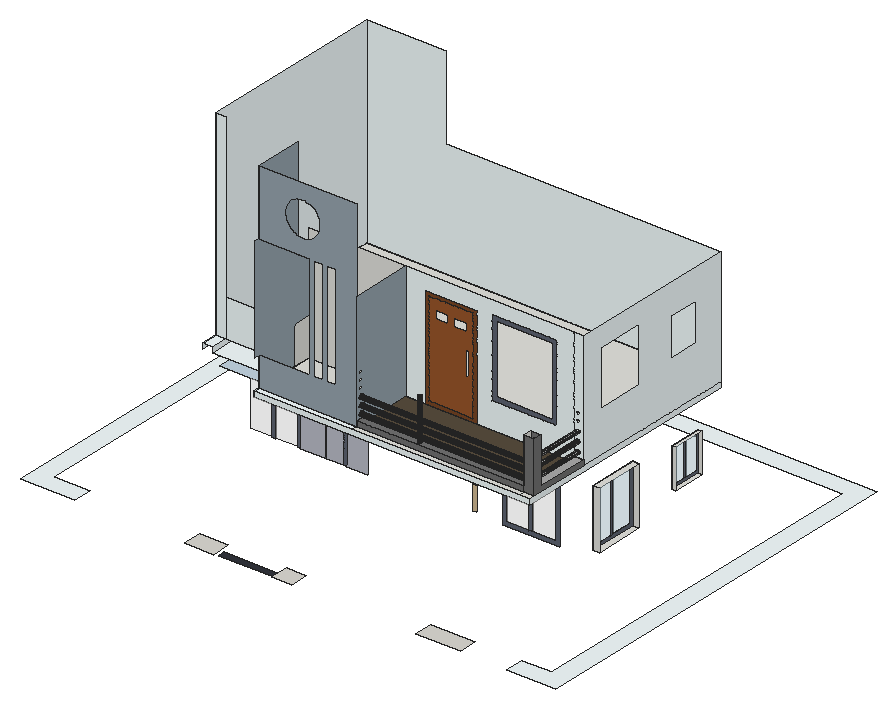
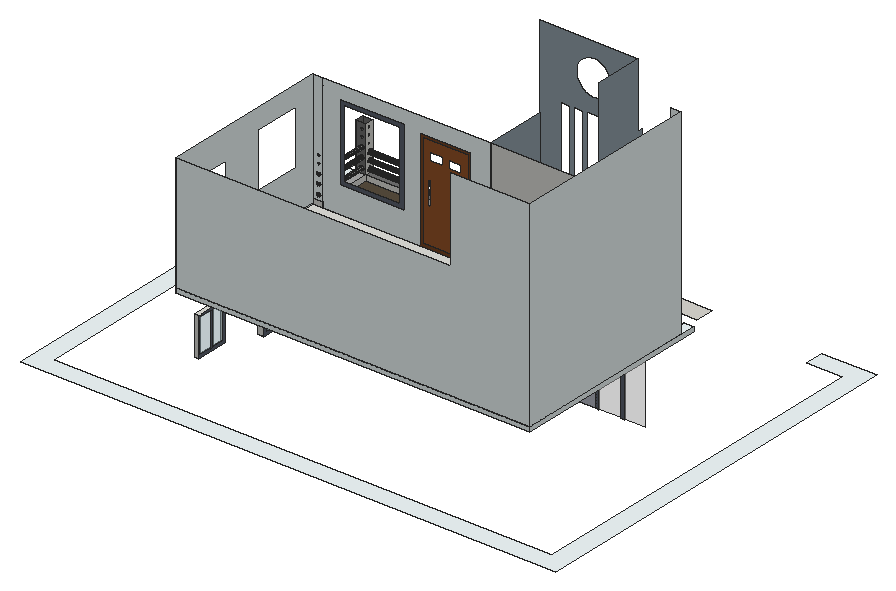
# SketchUp Ruby script. Lengths in inches.
U = 1.inch
M = Sketchup.active_model
def pt(a) = Geom::Point3d.new(a.map { |v| v * U })
def face(e, loops, mat)
  f = e.add_face(loops[0].map { |a| pt(a) })
  loops[1..].each { |l| e.add_face(l.map { |a| pt(a) }).erase! }
  f.material = f.back_material = mat if mat
  f
end
# faces: each face lists its corners as indices into pts; further lists are holes
def faces(e, pts, list, mat = nil) = list.each { |f| face(e, (f[0].is_a?(Array) ? f : [f]).map { |l| l.map { |i| pts[i] } }, mat) }
# xy, xz, yz: faces in a plane at the given z, y or x. An outline is a flat list of corners, or four numbers for a rectangle; further outlines are holes
def ring(l) = l.size == 4 ? [[l[0], l[1]], [l[2], l[1]], [l[2], l[3]], [l[0], l[3]]] : l.each_slice(2).to_a
def flat(e, list, mat, &to3) = list.each { |f| face(e, (f[0].is_a?(Array) ? f : [f]).map { |l| ring(l).map { |u, v| to3.(u, v) } }, mat) }
def xy(e, z, list, mat = nil) = flat(e, list, mat) { |x, y| [x, y, z] }
def xz(e, y, list, mat = nil) = flat(e, list, mat) { |x, z| [x, y, z] }
def yz(e, x, list, mat = nil) = flat(e, list, mat) { |y, z| [x, y, z] }
def lines(e, pts, list) = list.each { |a, b| e.add_line(pt(pts[a]), pt(pts[b])) }
# prism: a flat outline (further loops are holes) pulled along v
def prism(e, loops, v, mat = nil)
  f = face(e, loops, mat); d = Geom::Vector3d.new(v.map { |x| x * U })
  f.pushpull(f.normal.samedirection?(d) ? d.length : -d.length)
end
def box(e, o, s, mat = nil) = prism(e, [[o, [o[0] + s[0], o[1], o[2]], [o[0] + s[0], o[1] + s[1], o[2]], [o[0], o[1] + s[1], o[2]]]], [0, 0, s[2]], mat)
def at(x, y, z, deg = 0) = Geom::Transformation.translation(pt([x, y, z])) * Geom::Transformation.rotation(ORIGIN, Z_AXIS, deg.degrees)
def axes(o, x, y, z) = Geom::Transformation.new([*x, 0, *y, 0, *z, 0, *pt(o).to_a, 1])
def part(name) = M.definitions.add(name)
# library, detail: a bought-in or finely detailed component or shape, given as its bounding box
def library(name, o, s) = part(name).tap { |d| box(d.entities, o, s) }
def detail(e, o, s) = box(e.add_group.entities, o, s)
def put(e, d, t, mat = nil) = e.add_instance(d, t).tap { |i| i.material = mat if mat }
def group(e, t, mat = nil) = e.add_group.tap { |g| g.transformation = t; g.material = mat if mat }.entities
root = M.entities
M.materials.add("[Blinds Roman Hobbled Blue]").color = [187, 189, 201]
M.materials.add("[Carpet Diamond Olive]").color = [87, 77, 61]
M.materials.add("[Color M03]").color = [170, 170, 170]
M.materials.add("[Color M05]").color = [114, 114, 114]
M.materials.add("[Formica Beige]").color = [211, 187, 149]
M.materials.add("[Formica Graystone]").color = [229, 224, 207]
M.materials.add("[Formica Laminate Dark]").color = [95, 101, 114]
M.materials.add("[Formica Laminate Dark]1").color = [50, 53, 60]
M.materials.add("[Terrazzo Light Blue]").color = [151, 165, 175]
M.materials.add("[Terrazzo Light Blue]1").color = [196, 214, 227]
M.materials.add("[Terrazzo Tile Light]").color = [219, 217, 210]
M.materials.add("[Translucent Glass Gray]").color = [242, 242, 242]
M.materials["[Translucent Glass Gray]"].alpha = 0.5
M.materials.add("[Translucent Glass Safety]").color = [204, 235, 244]
M.materials["[Translucent Glass Safety]"].alpha = 0.5
M.materials.add("[White Subway Tile]").color = [243, 252, 253]
M.materials.add("[White Subway Tile]1").color = [243, 252, 253]
M.materials.add("[Wood Cherry Original]").color = [152, 86, 42]
M.materials.add("[Wood Veneer 01]").color = [120, 70, 37]
xy(root,402.23,[[1357.59,44.85,1765.91,92.78]],"[Formica Laminate Dark]1")
xy(root,402.84,[[2922.36,1375.57,2968.68,1724.7]])
xy(root,429.3125,[[1157.35,0,1357.59,129.42],[1765.91,0,1905.75,129.42],[2778.47,0,3092.67,129.42]],"[Terrazzo Tile Light]")
xy(root,429.3125,[[0,0,383.65,0,383.65,129.42,129.42,129.42,129.42,2686.64,3633.2,2686.64,3633.2,129.42,3421.78,129.42,3421.78,0,3762.625,0,3762.625,2816.0625,0,2816.0625]],"[White Subway Tile]1")
xy(root,498.46,[[2941.74,2046.63,2968.68,2278.38]])
xy(root,771.33,[[2941.74,2046.63,2968.68,2278.38]])
xy(root,809.34,[[2922.36,1375.57,2968.68,1724.7]])
xy(root,905.79,[[594.7,1008.89,1485.01,1239.01]],"[Terrazzo Light Blue]1")
xy(root,973.375,[[1034.97,761.77,1522.59,1008.89],[1522.59,761.77,1717.43,803.71],[2898.76,761.77,2968.68,803.71],[1034.97,1008.89,1522.59,1008.89,1522.59,1933.89,547.35,1933.89,547.35,1239.01,1034.97,1239.01],[1717.43,1239.01,2898.76,1933.89]])
xy(root,973.375,[[1717.43,761.77,2898.76,1239.01]],"[Terrazzo Light Blue]1")
xy(root,973.375,[[547.35,1008.89,1034.97,1239.01]],"[White Subway Tile]")
xy(root,1009.375,[[1720.33,761.77,2898.76,803.71],[2898.76,761.77,2968.68,803.71],[1034.97,803.71,1720.33,1239.01],[1720.33,803.71,1720.33,859.31,2898.76,859.31,2898.76,1239.01,2968.68,1239.01,2968.68,803.71],[477.43,1118.14,477.43,2442.87,2968.68,2442.87,2968.68,1239.01,547.35,1239.01,547.35,1118.14],
  [547.35,1118.14,1034.97,1239.01]])
xy(root,1009.375,[[1720.33,859.31,2898.76,1239.01]],"[Carpet Diamond Olive]")
xy(root,1009.375,[[1034.97,761.77,1720.33,803.71],[477.43,1008.89,547.35,1118.14]],"[White Subway Tile]")
xy(root,1046.4375,[[2140.61,820.84,2137.6,821.24,2134.79,822.4,2132.39,824.25,2130.54,826.66,2129.38,829.46,2128.98,832.47,2129.38,835.48,2130.54,838.28,2132.39,840.69,2134.79,842.54,2137.6,843.7,2140.61,844.09,2143.62,843.7,2146.42,842.54,2148.83,840.69,2150.67,838.28,2151.84,835.48,2152.23,832.47,2151.84,829.46,2150.67,826.66,2148.83,824.25,2146.42,822.4,2143.62,821.24]])
xy(root,1046.4375,[[2898.76,859.31,2968.68,1239.01]],"[Color M03]")
xy(root,1046.4375,[[[1720.33,803.71,2898.76,859.31],[2140.61,820.84,2137.6,821.24,2134.79,822.4,2132.39,824.25,2130.54,826.66,2129.38,829.46,2128.98,832.47,2129.38,835.48,2130.54,838.28,2132.39,840.69,2134.79,842.54,2137.6,843.7,2140.61,844.09,2143.62,843.7,2146.42,842.54,2148.83,840.69,2150.67,838.28,2151.84,835.48,2152.23,832.47,2151.84,829.46,2150.67,826.66,2148.83,824.25,2146.42,822.4,2143.62,821.24]]],"[Color M05]")
xz(root,761.77,[[1034.97,973.375,2968.68,1009.375]],"[White Subway Tile]")
xz(root,803.71,[[1720.33,1009.375,2898.76,1046.4375],[2898.76,1009.375,2968.68,1369.75]],"[Color M05]")
xz(root,803.71,[[[1034.97,1009.375,1720.33,1009.375,1720.33,2410.6875,1034.97,2410.6875,1034.97,1949.53,1389.66,1949.53,1389.66,1217.33,1034.97,1217.33],[1341.18,2057.61,1328.27,2058.29,1315.51,2060.3125,1303.02,2063.66,1290.95,2068.29,1279.43,2074.16,1268.59,2081.2,1258.55,2089.33,1249.4,2098.47,1241.27,2108.52,1234.23,2119.36,1228.36,2130.88,1223.73,2142.95,1220.38,2155.43,1218.36,2168.2,1217.68,2181.11,1218.36,2194.02,1220.38,2206.79,1223.73,2219.28,1228.36,2231.34,1234.23,2242.86,1241.27,2253.7,1249.4,2263.75,1258.55,2272.89,1268.59,2281.03,1279.43,2288.07,1290.95,2293.93,1303.02,2298.57,1315.51,2301.91,1328.27,2303.94,1341.18,2304.61,1354.09,2303.94,1366.86,2301.91,1379.35,2298.57,1391.42,2293.93,1402.93,2288.07,1413.77,2281.03,1423.82,2272.89,1432.96,2263.75,1441.1,2253.7,1448.14,2242.86,1454.01,2231.34,1458.64,2219.28,1461.98,2206.79,1464.01,2194.02,1464.68,2181.11,1464.01,2168.2,1461.98,2155.43,1458.64,2142.95,1454.01,2130.88,1448.14,2119.36,1441.1,2108.52,1432.96,2098.47,1423.82,2089.33,1413.77,2081.2,1402.93,2074.16,1391.42,2068.29,1379.35,2063.66,1366.86,2060.3125,1354.09,2058.29],[1421.94,1217.36,1482.63,1947.36],[1511.44,1217.36,1572.13,1947.36]]],"[Terrazzo Light Blue]")
xz(root,859.31,[[1720.33,1009.375,2898.76,1046.4375],[2927.58,1067.59,2930.84,1068.02,2933.87,1069.27,2936.47,1071.27,2938.46,1073.87,2939.72,1076.9,2940.15,1080.15,2939.72,1083.4,2938.46,1086.43,2936.47,1089.03,2933.87,1091.03,2930.84,1092.29,2927.58,1092.71,2924.33,1092.29,2921.3,1091.03,2918.7,1089.03,2916.7,1086.43,2915.45,1083.4,2915.02,1080.15,2915.45,1076.9,2916.7,1073.87,2918.7,1071.27,2921.3,1069.27,2924.33,1068.02],[2927.58,1135.59,2930.84,1136.02,2933.87,1137.27,2936.47,1139.27,2938.46,1141.87,2939.72,1144.9,2940.15,1148.15,2939.72,1151.4,2938.46,1154.43,2936.47,1157.03,2933.87,1159.03,2930.84,1160.29,2927.58,1160.71,2924.33,1160.29,2921.3,1159.03,2918.7,1157.03,2916.7,1154.43,2915.45,1151.4,2915.02,1148.15,2915.45,1144.9,2916.7,1141.87,2918.7,1139.27,2921.3,1137.27,2924.33,1136.02],[2927.58,1200.78,2930.84,1201.2,2933.87,1202.46,2936.47,1204.46,2938.46,1207.06,2939.72,1210.09,2940.15,1213.34,2939.72,1216.59,2938.46,1219.62,2936.47,1222.22,2933.87,1224.22,2930.84,1225.47,2927.58,1225.9,2924.33,1225.47,2921.3,1224.22,2918.7,1222.22,2916.7,1219.62,2915.45,1216.59,2915.02,1213.34,2915.45,1210.09,2916.7,1207.06,2918.7,1204.46,2921.3,1202.46,2924.33,1201.2]])
xz(root,859.31,[[[2898.76,1046.4375,2968.68,1369.75],[2927.58,1316.03,2930.84,1316.45,2933.87,1317.71,2936.47,1319.71,2938.46,1322.31,2939.72,1325.34,2940.15,1328.59,2939.72,1331.84,2938.46,1334.87,2936.47,1337.47,2933.87,1339.47,2930.84,1340.72,2927.58,1341.15,2924.33,1340.72,2921.3,1339.47,2918.7,1337.47,2916.7,1334.87,2915.45,1331.84,2915.02,1328.59,2915.45,1325.34,2916.7,1322.31,2918.7,1319.71,2921.3,1317.71,2924.33,1316.45],[2927.58,1067.59,2930.84,1068.02,2933.87,1069.27,2936.47,1071.27,2938.46,1073.87,2939.72,1076.9,2940.15,1080.15,2939.72,1083.4,2938.46,1086.43,2936.47,1089.03,2933.87,1091.03,2930.84,1092.29,2927.58,1092.71,2924.33,1092.29,2921.3,1091.03,2918.7,1089.03,2916.7,1086.43,2915.45,1083.4,2915.02,1080.15,2915.45,1076.9,2916.7,1073.87,2918.7,1071.27,2921.3,1069.27,2924.33,1068.02],[2927.58,1264.46,2930.84,1264.89,2933.87,1266.15,2936.47,1268.14,2938.46,1270.75,2939.72,1273.77,2940.15,1277.03,2939.72,1280.28,2938.46,1283.31,2936.47,1285.91,2933.87,1287.91,2930.84,1289.16,2927.58,1289.59,2924.33,1289.16,2921.3,1287.91,2918.7,1285.91,2916.7,1283.31,2915.45,1280.28,2915.02,1277.03,2915.45,1273.77,2916.7,1270.75,2918.7,1268.14,2921.3,1266.15,2924.33,1264.89],[2927.58,1135.59,2930.84,1136.02,2933.87,1137.27,2936.47,1139.27,2938.46,1141.87,2939.72,1144.9,2940.15,1148.15,2939.72,1151.4,2938.46,1154.43,2936.47,1157.03,2933.87,1159.03,2930.84,1160.29,2927.58,1160.71,2924.33,1160.29,2921.3,1159.03,2918.7,1157.03,2916.7,1154.43,2915.45,1151.4,2915.02,1148.15,2915.45,1144.9,2916.7,1141.87,2918.7,1139.27,2921.3,1137.27,2924.33,1136.02],[2927.58,1200.78,2930.84,1201.2,2933.87,1202.46,2936.47,1204.46,2938.46,1207.06,2939.72,1210.09,2940.15,1213.34,2939.72,1216.59,2938.46,1219.62,2936.47,1222.22,2933.87,1224.22,2930.84,1225.47,2927.58,1225.9,2924.33,1225.47,2921.3,1224.22,2918.7,1222.22,2916.7,1219.62,2915.45,1216.59,2915.02,1213.34,2915.45,1210.09,2916.7,1207.06,2918.7,1204.46,2921.3,1202.46,2924.33,1201.2]]],"[Color M05]")
xz(root,1118.14,[[477.43,1009.375,547.35,2410.6875],[547.35,1009.375,1034.97,1272.1]],"[White Subway Tile]")
xz(root,1239.01,[[547.35,973.375,1034.97,1009.375],[1034.97,1009.375,1720.33,1828.125],[2898.76,1009.375,2968.68,1046.4375]])
xz(root,1239.01,[[981.69,419.96,1149.58,873.24],[1165.1875,419.96,1280.47,873.24],[1305.85,419.96,1452.47,873.24]],"[Blinds Roman Hobbled Blue]")
xz(root,1239.01,[[2190.67,454.58,2217.05,620.33]],"[Formica Beige]")
xz(root,1239.01,[[2125.16,693.23,2217.66,761.05],[1985.88,705.68,2074.875,760.68]],"[Formica Graystone]")
xz(root,1239.01,[[778.16,419.96,803.87,873.24],[957.16,419.96,981.69,873.24],[1149.58,419.96,1165.1875,873.24],[1280.47,419.96,1305.85,873.24],[[2398.08,439.46,2800.45,879.09],[2425.17,466.55,2773.37,852]],
  [2585.66,466.55,2609.16,852],[[2322.55,1192.6,2780.61,1737.72],[2353.98,1224.02,2749.1875,1706.3]]],"[Formica Laminate Dark]")
xz(root,1239.01,[[627.24,419.96,778.16,873.24],[803.87,419.96,957.16,873.24],[2425.17,466.55,2585.66,852],[2609.16,466.55,2773.37,852]],"[Translucent Glass Gray]")
xz(root,1239.01,[[[1720.33,1009.375,1856.64,1009.375,1856.64,1722.125,2215.15,1722.125,2215.15,1009.375,2898.76,1009.375,2898.76,1828.125,1720.33,1828.125],[2322.55,1192.6,2780.61,1737.72]],[[2898.76,1046.4375,2968.68,1828.125],[2927.58,1316.03,2924.33,1316.45,2921.3,1317.71,2918.7,1319.71,2916.7,1322.31,2915.45,1325.34,2915.02,1328.59,2915.45,1331.84,2916.7,1334.87,2918.7,1337.47,2921.3,1339.47,2924.33,1340.72,2927.58,1341.15,2930.84,1340.72,2933.87,1339.47,2936.47,1337.47,2938.46,1334.87,2939.72,1331.84,2940.15,1328.59,2939.72,1325.34,2938.46,1322.31,2936.47,1319.71,2933.87,1317.71,2930.84,1316.45],[2927.58,1264.46,2924.33,1264.89,2921.3,1266.15,2918.7,1268.14,2916.7,1270.75,2915.45,1273.77,2915.02,1277.03,2915.45,1280.28,2916.7,1283.31,2918.7,1285.91,2921.3,1287.91,2924.33,1289.16,2927.58,1289.59,2930.84,1289.16,2933.87,1287.91,2936.47,1285.91,2938.46,1283.31,2939.72,1280.28,2940.15,1277.03,2939.72,1273.77,2938.46,1270.75,2936.47,1268.14,2933.87,1266.15,2930.84,1264.89],[2927.58,1200.78,2924.33,1201.2,2921.3,1202.46,2918.7,1204.46,2916.7,1207.06,2915.45,1210.09,2915.02,1213.34,2915.45,1216.59,2916.7,1219.62,2918.7,1222.22,2921.3,1224.22,2924.33,1225.47,2927.58,1225.9,2930.84,1225.47,2933.87,1224.22,2936.47,1222.22,2938.46,1219.62,2939.72,1216.59,2940.15,1213.34,2939.72,1210.09,2938.46,1207.06,2936.47,1204.46,2933.87,1202.46,2930.84,1201.2],[2927.58,1135.59,2924.33,1136.02,2921.3,1137.27,2918.7,1139.27,2916.7,1141.87,2915.45,1144.9,2915.02,1148.15,2915.45,1151.4,2916.7,1154.43,2918.7,1157.03,2921.3,1159.03,2924.33,1160.29,2927.58,1160.71,2930.84,1160.29,2933.87,1159.03,2936.47,1157.03,2938.46,1154.43,2939.72,1151.4,2940.15,1148.15,2939.72,1144.9,2938.46,1141.87,2936.47,1139.27,2933.87,1137.27,2930.84,1136.02],[2927.58,1067.59,2924.33,1068.02,2921.3,1069.27,2918.7,1071.27,2916.7,1073.87,2915.45,1076.9,2915.02,1080.15,2915.45,1083.4,2916.7,1086.43,2918.7,1089.03,2921.3,1091.03,2924.33,1092.29,2927.58,1092.71,2930.84,1092.29,2933.87,1091.03,2936.47,1089.03,2938.46,1086.43,2939.72,1083.4,2940.15,1080.15,2939.72,1076.9,2938.46,1073.87,2936.47,1071.27,2933.87,1069.27,2930.84,1068.02]]],"[White Subway Tile]")
xz(root,1239.01,[[[1880.3,1033.03,2191.5,1698.47],[1925.5625,1566.2,2014.55,1621.2],[2058.375,1566.2,2147.37,1621.2],[2136.34,1281.23,2162.72,1446.98]]],"[Wood Cherry Original]")
xz(root,1239.01,[[[1856.64,1009.375,2215.15,1722.125],[1880.3,1033.03,2191.5,1698.47]]],"[Wood Veneer 01]")
xz(root,1375.57,[[2922.36,402.84,2968.68,809.34]])
xz(root,1724.7,[[2922.36,402.84,2968.68,809.34]])
xz(root,2046.63,[[2941.74,498.46,2968.68,771.33]])
xz(root,2278.38,[[2941.74,498.46,2968.68,771.33]])
xz(root,2442.87,[[477.43,973.375,2968.68,1009.375],[477.43,1009.375,477.43,2410.6875,1034.97,2410.6875,1034.97,1828.125,2968.68,1828.125,2968.68,1009.375]],"[White Subway Tile]")
yz(root,477.43,[[1008.89,973.375,2442.87,1009.375],[1118.14,1009.375,2442.87,2410.6875]],"[White Subway Tile]")
yz(root,547.35,[[1008.89,973.375,1239.01,1009.375]],"[White Subway Tile]")
yz(root,1034.97,[[1118.14,1009.375,1239.01,1272.1]])
yz(root,1034.97,[[803.71,1009.375,803.71,1217.33,767.89,1217.33,767.89,1949.53,803.71,1949.53,803.71,2410.6875,1146.14,2410.6875,1146.14,1690.66,1239.01,1690.66,1239.01,1272.1,1118.14,1272.1,1118.14,1009.375]],"[Terrazzo Light Blue]")
yz(root,1034.97,[[761.77,973.375,1239.01,1009.375]],"[White Subway Tile]")
yz(root,1720.33,[[803.71,1009.375,859.31,1046.4375]])
yz(root,1720.33,[[[859.31,1009.375,1239.01,1009.375,1239.01,1828.125,803.71,1828.125,803.71,1046.4375,859.31,1046.4375],[834.19,1325.79,830.94,1326.22,827.91,1327.47,825.3125,1329.47,823.32,1332.07,822.06,1335.1,821.63,1338.35,822.06,1341.6,823.32,1344.63,825.3125,1347.24,827.91,1349.23,830.94,1350.49,834.19,1350.92,837.45,1350.49,840.48,1349.23,843.08,1347.24,845.07,1344.63,846.33,1341.6,846.76,1338.35,846.33,1335.1,845.07,1332.07,843.08,1329.47,840.48,1327.47,837.45,1326.22],[834.19,1277.73,830.94,1278.16,827.91,1279.41,825.3125,1281.41,823.32,1284.01,822.06,1287.04,821.63,1290.29,822.06,1293.54,823.32,1296.57,825.3125,1299.17,827.91,1301.17,830.94,1302.43,834.19,1302.85,837.45,1302.43,840.48,1301.17,843.08,1299.17,845.07,1296.57,846.33,1293.54,846.76,1290.29,846.33,1287.04,845.07,1284.01,843.08,1281.41,840.48,1279.41,837.45,1278.16],[834.19,1224.6,830.94,1225.03,827.91,1226.29,825.3125,1228.28,823.32,1230.88,822.06,1233.91,821.63,1237.17,822.06,1240.42,823.32,1243.45,825.3125,1246.05,827.91,1248.05,830.94,1249.3,834.19,1249.73,837.45,1249.3,840.48,1248.05,843.08,1246.05,845.07,1243.45,846.33,1240.42,846.76,1237.17,846.33,1233.91,845.07,1230.88,843.08,1228.28,840.48,1226.29,837.45,1225.03],[834.19,1172.92,830.94,1173.34,827.91,1174.6,825.3125,1176.6,823.32,1179.2,822.06,1182.23,821.63,1185.48,822.06,1188.73,823.32,1191.76,825.3125,1194.36,827.91,1196.36,830.94,1197.61,834.19,1198.04,837.45,1197.61,840.48,1196.36,843.08,1194.36,845.07,1191.76,846.33,1188.73,846.76,1185.48,846.33,1182.23,845.07,1179.2,843.08,1176.6,840.48,1174.6,837.45,1173.34],[834.19,1120.17,830.94,1120.59,827.91,1121.85,825.3125,1123.85,823.32,1126.45,822.06,1129.48,821.63,1132.73,822.06,1135.98,823.32,1139.01,825.3125,1141.61,827.91,1143.61,830.94,1144.86,834.19,1145.29,837.45,1144.86,840.48,1143.61,843.08,1141.61,845.07,1139.01,846.33,1135.98,846.76,1132.73,846.33,1129.48,845.07,1126.45,843.08,1123.85,840.48,1121.85,837.45,1120.59],[834.19,1065.04,830.94,1065.47,827.91,1066.72,825.3125,1068.72,823.32,1071.32,822.06,1074.35,821.63,1077.6,822.06,1080.85,823.32,1083.88,825.3125,1086.49,827.91,1088.48,830.94,1089.74,834.19,1090.17,837.45,1089.74,840.48,1088.48,843.08,1086.49,845.07,1083.88,846.33,1080.85,846.76,1077.6,846.33,1074.35,845.07,1071.32,843.08,1068.72,840.48,1066.72,837.45,1065.47]]],"[Terrazzo Light Blue]")
yz(root,2898.76,[[859.31,1009.375,1239.01,1046.4375],[[803.71,1046.4375,859.31,1369.75],[834.19,1325.79,837.45,1326.22,840.48,1327.47,843.08,1329.47,845.07,1332.07,846.33,1335.1,846.76,1338.35,846.33,1341.6,845.07,1344.63,843.08,1347.24,840.48,1349.23,837.45,1350.49,834.19,1350.92,830.94,1350.49,827.91,1349.23,825.3125,1347.24,823.32,1344.63,822.06,1341.6,821.63,1338.35,822.06,1335.1,823.32,1332.07,825.3125,1329.47,827.91,1327.47,830.94,1326.22],[834.19,1065.04,837.45,1065.47,840.48,1066.72,843.08,1068.72,845.07,1071.32,846.33,1074.35,846.76,1077.6,846.33,1080.85,845.07,1083.88,843.08,1086.49,840.48,1088.48,837.45,1089.74,834.19,1090.17,830.94,1089.74,827.91,1088.48,825.3125,1086.49,823.32,1083.88,822.06,1080.85,821.63,1077.6,822.06,1074.35,823.32,1071.32,825.3125,1068.72,827.91,1066.72,830.94,1065.47],[834.19,1277.73,837.45,1278.16,840.48,1279.41,843.08,1281.41,845.07,1284.01,846.33,1287.04,846.76,1290.29,846.33,1293.54,845.07,1296.57,843.08,1299.17,840.48,1301.17,837.45,1302.43,834.19,1302.85,830.94,1302.43,827.91,1301.17,825.3125,1299.17,823.32,1296.57,822.06,1293.54,821.63,1290.29,822.06,1287.04,823.32,1284.01,825.3125,1281.41,827.91,1279.41,830.94,1278.16],[834.19,1120.17,837.45,1120.59,840.48,1121.85,843.08,1123.85,845.07,1126.45,846.33,1129.48,846.76,1132.73,846.33,1135.98,845.07,1139.01,843.08,1141.61,840.48,1143.61,837.45,1144.86,834.19,1145.29,830.94,1144.86,827.91,1143.61,825.3125,1141.61,823.32,1139.01,822.06,1135.98,821.63,1132.73,822.06,1129.48,823.32,1126.45,825.3125,1123.85,827.91,1121.85,830.94,1120.59],[834.19,1224.6,837.45,1225.03,840.48,1226.29,843.08,1228.28,845.07,1230.88,846.33,1233.91,846.76,1237.17,846.33,1240.42,845.07,1243.45,843.08,1246.05,840.48,1248.05,837.45,1249.3,834.19,1249.73,830.94,1249.3,827.91,1248.05,825.3125,1246.05,823.32,1243.45,822.06,1240.42,821.63,1237.17,822.06,1233.91,823.32,1230.88,825.3125,1228.28,827.91,1226.29,830.94,1225.03],[834.19,1172.92,837.45,1173.34,840.48,1174.6,843.08,1176.6,845.07,1179.2,846.33,1182.23,846.76,1185.48,846.33,1188.73,845.07,1191.76,843.08,1194.36,840.48,1196.36,837.45,1197.61,834.19,1198.04,830.94,1197.61,827.91,1196.36,825.3125,1194.36,823.32,1191.76,822.06,1188.73,821.63,1185.48,822.06,1182.23,823.32,1179.2,825.3125,1176.6,827.91,1174.6,830.94,1173.34]],[834.19,1065.04,837.45,1065.47,840.48,1066.72,843.08,1068.72,845.07,1071.32,846.33,1074.35,846.76,1077.6,846.33,1080.85,845.07,1083.88,843.08,1086.49,840.48,1088.48,837.45,1089.74,834.19,1090.17,830.94,1089.74,827.91,1088.48,825.3125,1086.49,823.32,1083.88,822.06,1080.85,821.63,1077.6,822.06,1074.35,823.32,1071.32,825.3125,1068.72,827.91,1066.72,830.94,1065.47],[834.19,1120.17,837.45,1120.59,840.48,1121.85,843.08,1123.85,845.07,1126.45,846.33,1129.48,846.76,1132.73,846.33,1135.98,845.07,1139.01,843.08,1141.61,840.48,1143.61,837.45,1144.86,834.19,1145.29,830.94,1144.86,827.91,1143.61,825.3125,1141.61,823.32,1139.01,822.06,1135.98,821.63,1132.73,822.06,1129.48,823.32,1126.45,825.3125,1123.85,827.91,1121.85,830.94,1120.59],[834.19,1172.92,837.45,1173.34,840.48,1174.6,843.08,1176.6,845.07,1179.2,846.33,1182.23,846.76,1185.48,846.33,1188.73,845.07,1191.76,843.08,1194.36,840.48,1196.36,837.45,1197.61,834.19,1198.04,830.94,1197.61,827.91,1196.36,825.3125,1194.36,823.32,1191.76,822.06,1188.73,821.63,1185.48,822.06,1182.23,823.32,1179.2,825.3125,1176.6,827.91,1174.6,830.94,1173.34]])
yz(root,2922.36,[[[1375.57,402.84,1724.7,809.34],[1394.9,422.17,1705.37,790.01]],[1537.67,422.17,1555.72,790.01]],"[Formica Laminate Dark]")
yz(root,2922.36,[[1394.9,422.17,1537.67,790.01],[1555.72,422.17,1705.37,790.01]],"[Translucent Glass Safety]")
yz(root,2941.74,[[[2046.63,498.46,2278.38,771.33],[2064.02,515.84,2261,753.95]],[2153.63,515.84,2169.77,753.95]],"[Formica Laminate Dark]")
yz(root,2941.74,[[2064.02,515.84,2153.63,753.95],[2169.77,515.84,2261,753.95]],"[Translucent Glass Safety]")
yz(root,2968.68,[[803.71,1009.375,1239.01,1009.375,1239.01,1046.4375,859.31,1046.4375,859.31,1369.75,803.71,1369.75]],"[Color M05]")
yz(root,2968.68,[[761.77,973.375,2442.87,1009.375],[[1239.01,1009.375,2442.87,1828.125],[1390.76,1302.22,1726.13,1686.6],[2002.64,1348.11,2223.02,1615.93]]],"[White Subway Tile]")
p = [[2137.6,821.24,1046.4375],[2140.61,820.84,1046.4375],[2140.61,820.84,1339.25],[2137.6,821.24,1339.25],[2143.62,821.24,1046.4375],[2143.62,821.24,1339.25],
  [2134.79,822.4,1046.4375],[2134.79,822.4,1339.25],[2146.42,822.4,1046.4375],[2146.42,822.4,1339.25],[2132.39,824.25,1046.4375],[2132.39,824.25,1339.25],
  [2148.83,824.25,1046.4375],[2148.83,824.25,1339.25],[2130.54,826.66,1046.4375],[2130.54,826.66,1339.25],[2150.67,826.66,1046.4375],[2150.67,826.66,1339.25],
  [2129.38,829.46,1046.4375],[2129.38,829.46,1339.25],[2151.84,829.46,1046.4375],[2151.84,829.46,1339.25],[2128.98,832.47,1046.4375],[2128.98,832.47,1339.25],
  [2152.23,832.47,1046.4375],[2152.23,832.47,1339.25],[2129.38,835.48,1046.4375],[2129.38,835.48,1339.25],[2151.84,835.48,1046.4375],[2151.84,835.48,1339.25],
  [2130.54,838.28,1046.4375],[2130.54,838.28,1339.25],[2150.67,838.28,1046.4375],[2150.67,838.28,1339.25],[2132.39,840.69,1046.4375],[2132.39,840.69,1339.25],
  [2148.83,840.69,1046.4375],[2148.83,840.69,1339.25],[2134.79,842.54,1046.4375],[2134.79,842.54,1339.25],[2146.42,842.54,1046.4375],[2146.42,842.54,1339.25],
  [2137.6,843.7,1046.4375],[2137.6,843.7,1339.25],[2143.62,843.7,1046.4375],[2143.62,843.7,1339.25],[2140.61,844.09,1046.4375],[2140.61,844.09,1339.25],
  [2898.76,834.19,1065.04],[2898.76,830.94,1065.47],[1720.33,830.94,1065.47],[1720.33,834.19,1065.04],[2898.76,837.45,1065.47],[1720.33,837.45,1065.47],
  [2898.76,827.91,1066.72],[1720.33,827.91,1066.72],[2898.76,840.48,1066.72],[1720.33,840.48,1066.72],[2898.76,825.3125,1068.72],[1720.33,825.3125,1068.72],
  [2898.76,843.08,1068.72],[1720.33,843.08,1068.72],[2927.58,859.31,1067.59],[2924.33,859.31,1068.02],[2924.33,1239.01,1068.02],[2927.58,1239.01,1067.59],
  [2930.84,859.31,1068.02],[2930.84,1239.01,1068.02],[2921.3,859.31,1069.27],[2921.3,1239.01,1069.27],[2933.87,859.31,1069.27],[2933.87,1239.01,1069.27],
  [2898.76,823.32,1071.32],[1720.33,823.32,1071.32],[2898.76,845.07,1071.32],[1720.33,845.07,1071.32],[2918.7,859.31,1071.27],[2918.7,1239.01,1071.27],
  [2936.47,859.31,1071.27],[2936.47,1239.01,1071.27],[2898.76,822.06,1074.35],[1720.33,822.06,1074.35],[2898.76,846.33,1074.35],[1720.33,846.33,1074.35],
  [2916.7,859.31,1073.87],[2916.7,1239.01,1073.87],[2938.46,859.31,1073.87],[2938.46,1239.01,1073.87],[2915.45,859.31,1076.9],[2915.45,1239.01,1076.9],
  [2939.72,859.31,1076.9],[2939.72,1239.01,1076.9],[2898.76,821.63,1077.6],[1720.33,821.63,1077.6],[2898.76,846.76,1077.6],[1720.33,846.76,1077.6],
  [2915.02,859.31,1080.15],[2915.02,1239.01,1080.15],[2940.15,859.31,1080.15],[2940.15,1239.01,1080.15],[2898.76,822.06,1080.85],[1720.33,822.06,1080.85],
  [2898.76,846.33,1080.85],[1720.33,846.33,1080.85],[2915.45,859.31,1083.4],[2915.45,1239.01,1083.4],[2939.72,859.31,1083.4],[2939.72,1239.01,1083.4],
  [2898.76,823.32,1083.88],[1720.33,823.32,1083.88],[2898.76,845.07,1083.88],[1720.33,845.07,1083.88],[2916.7,859.31,1086.43],[2916.7,1239.01,1086.43],
  [2938.46,859.31,1086.43],[2938.46,1239.01,1086.43],[2898.76,825.3125,1086.49],[1720.33,825.3125,1086.49],[2898.76,843.08,1086.49],[1720.33,843.08,1086.49],
  [2918.7,859.31,1089.03],[2918.7,1239.01,1089.03],[2936.47,859.31,1089.03],[2936.47,1239.01,1089.03],[2898.76,827.91,1088.48],[1720.33,827.91,1088.48],
  [2898.76,840.48,1088.48],[1720.33,840.48,1088.48],[2898.76,830.94,1089.74],[1720.33,830.94,1089.74],[2898.76,837.45,1089.74],[1720.33,837.45,1089.74],
  [2921.3,859.31,1091.03],[2921.3,1239.01,1091.03],[2933.87,859.31,1091.03],[2933.87,1239.01,1091.03],[2898.76,834.19,1090.17],[1720.33,834.19,1090.17],
  [2924.33,859.31,1092.29],[2924.33,1239.01,1092.29],[2930.84,859.31,1092.29],[2930.84,1239.01,1092.29],[2927.58,859.31,1092.71],[2927.58,1239.01,1092.71],
  [2898.76,834.19,1120.17],[2898.76,830.94,1120.59],[1720.33,830.94,1120.59],[1720.33,834.19,1120.17],[2898.76,837.45,1120.59],[1720.33,837.45,1120.59],
  [2898.76,827.91,1121.85],[1720.33,827.91,1121.85],[2898.76,840.48,1121.85],[1720.33,840.48,1121.85],[2898.76,825.3125,1123.85],[1720.33,825.3125,1123.85],
  [2898.76,843.08,1123.85],[1720.33,843.08,1123.85],[2898.76,823.32,1126.45],[1720.33,823.32,1126.45],[2898.76,845.07,1126.45],[1720.33,845.07,1126.45],
  [2898.76,822.06,1129.48],[1720.33,822.06,1129.48],[2898.76,846.33,1129.48],[1720.33,846.33,1129.48],[2898.76,821.63,1132.73],[1720.33,821.63,1132.73],
  [2898.76,846.76,1132.73],[1720.33,846.76,1132.73],[2898.76,822.06,1135.98],[1720.33,822.06,1135.98],[2898.76,846.33,1135.98],[1720.33,846.33,1135.98],
  [2927.58,859.31,1135.59],[2924.33,859.31,1136.02],[2924.33,1239.01,1136.02],[2927.58,1239.01,1135.59],[2930.84,859.31,1136.02],[2930.84,1239.01,1136.02],
  [2898.76,823.32,1139.01],[1720.33,823.32,1139.01],[2898.76,845.07,1139.01],[1720.33,845.07,1139.01],[2921.3,859.31,1137.27],[2921.3,1239.01,1137.27],
  [2933.87,859.31,1137.27],[2933.87,1239.01,1137.27],[2918.7,859.31,1139.27],[2918.7,1239.01,1139.27],[2936.47,859.31,1139.27],[2936.47,1239.01,1139.27],
  [2898.76,825.3125,1141.61],[1720.33,825.3125,1141.61],[2898.76,843.08,1141.61],[1720.33,843.08,1141.61],[2916.7,859.31,1141.87],[2916.7,1239.01,1141.87],
  [2938.46,859.31,1141.87],[2938.46,1239.01,1141.87],[2898.76,827.91,1143.61],[1720.33,827.91,1143.61],[2898.76,840.48,1143.61],[1720.33,840.48,1143.61],
  [2915.45,859.31,1144.9],[2915.45,1239.01,1144.9],[2939.72,859.31,1144.9],[2939.72,1239.01,1144.9],[2898.76,830.94,1144.86],[1720.33,830.94,1144.86],
  [2898.76,837.45,1144.86],[1720.33,837.45,1144.86],[2898.76,834.19,1145.29],[1720.33,834.19,1145.29],[2915.02,859.31,1148.15],[2915.02,1239.01,1148.15],
  [2940.15,859.31,1148.15],[2940.15,1239.01,1148.15],[2915.45,859.31,1151.4],[2915.45,1239.01,1151.4],[2939.72,859.31,1151.4],[2939.72,1239.01,1151.4],
  [2916.7,859.31,1154.43],[2916.7,1239.01,1154.43],[2938.46,859.31,1154.43],[2938.46,1239.01,1154.43],[2918.7,859.31,1157.03],[2918.7,1239.01,1157.03],
  [2936.47,859.31,1157.03],[2936.47,1239.01,1157.03],[2921.3,859.31,1159.03],[2921.3,1239.01,1159.03],[2933.87,859.31,1159.03],[2933.87,1239.01,1159.03],
  [2924.33,859.31,1160.29],[2924.33,1239.01,1160.29],[2930.84,859.31,1160.29],[2930.84,1239.01,1160.29],[2927.58,859.31,1160.71],[2927.58,1239.01,1160.71],
  [2898.76,834.19,1172.92],[2898.76,830.94,1173.34],[1720.33,830.94,1173.34],[1720.33,834.19,1172.92],[2898.76,837.45,1173.34],[1720.33,837.45,1173.34],
  [2898.76,827.91,1174.6],[1720.33,827.91,1174.6],[2898.76,840.48,1174.6],[1720.33,840.48,1174.6],[2898.76,825.3125,1176.6],[1720.33,825.3125,1176.6],
  [2898.76,843.08,1176.6],[1720.33,843.08,1176.6],[2898.76,823.32,1179.2],[1720.33,823.32,1179.2],[2898.76,845.07,1179.2],[1720.33,845.07,1179.2],
  [2898.76,822.06,1182.23],[1720.33,822.06,1182.23],[2898.76,846.33,1182.23],[1720.33,846.33,1182.23],[2898.76,821.63,1185.48],[1720.33,821.63,1185.48],
  [2898.76,846.76,1185.48],[1720.33,846.76,1185.48],[2898.76,822.06,1188.73],[1720.33,822.06,1188.73],[2898.76,846.33,1188.73],[1720.33,846.33,1188.73],
  [2898.76,823.32,1191.76],[1720.33,823.32,1191.76],[2898.76,845.07,1191.76],[1720.33,845.07,1191.76],[2898.76,825.3125,1194.36],[1720.33,825.3125,1194.36],
  [2898.76,843.08,1194.36],[1720.33,843.08,1194.36],[2898.76,827.91,1196.36],[1720.33,827.91,1196.36],[2898.76,840.48,1196.36],[1720.33,840.48,1196.36],
  [2898.76,830.94,1197.61],[1720.33,830.94,1197.61],[2898.76,837.45,1197.61],[1720.33,837.45,1197.61],[2898.76,834.19,1198.04],[1720.33,834.19,1198.04],
  [2927.58,859.31,1200.78],[2924.33,859.31,1201.2],[2924.33,1239.01,1201.2],[2927.58,1239.01,1200.78],[2930.84,859.31,1201.2],[2930.84,1239.01,1201.2],
  [2921.3,859.31,1202.46],[2921.3,1239.01,1202.46],[2933.87,859.31,1202.46],[2933.87,1239.01,1202.46],[2918.7,859.31,1204.46],[2918.7,1239.01,1204.46],
  [2936.47,859.31,1204.46],[2936.47,1239.01,1204.46],[2916.7,859.31,1207.06],[2916.7,1239.01,1207.06],[2938.46,859.31,1207.06],[2938.46,1239.01,1207.06],
  [2915.45,859.31,1210.09],[2915.45,1239.01,1210.09],[2939.72,859.31,1210.09],[2939.72,1239.01,1210.09],[2915.02,859.31,1213.34],[2915.02,1239.01,1213.34],
  [2940.15,859.31,1213.34],[2940.15,1239.01,1213.34],[2915.45,859.31,1216.59],[2915.45,1239.01,1216.59],[2939.72,859.31,1216.59],[2939.72,1239.01,1216.59],
  [2916.7,859.31,1219.62],[2916.7,1239.01,1219.62],[2938.46,859.31,1219.62],[2938.46,1239.01,1219.62]]
faces(root,p,[[0,1,2,3],[1,4,5,2],[6,0,3,7],[4,8,9,5],[10,6,7,11],[8,12,13,9],[14,10,11,15],[12,16,17,13],
  [18,14,15,19],[16,20,21,17],[22,18,19,23],[20,24,25,21],[26,22,23,27],[24,28,29,25],[30,26,27,31],[28,32,33,29],
  [34,30,31,35],[32,36,37,33],[38,34,35,39],[36,40,41,37],[42,38,39,43],[40,44,45,41],[46,42,43,47],[44,46,47,45],
  [48,49,50,51],[52,48,51,53],[49,54,55,50],[56,52,53,57],[54,58,59,55],[60,56,57,61],[62,63,64,65],[66,62,65,67],
  [63,68,69,64],[70,66,67,71],[58,72,73,59],[74,60,61,75],[68,76,77,69],[78,70,71,79],[72,80,81,73],[82,74,75,83],
  [76,84,85,77],[86,78,79,87],[84,88,89,85],[90,86,87,91],[80,92,93,81],[94,82,83,95],[88,96,97,89],[98,90,91,99],
  [92,100,101,93],[102,94,95,103],[96,104,105,97],[106,98,99,107],[100,108,109,101],[110,102,103,111],[104,112,113,105],[114,106,107,115],
  [108,116,117,109],[118,110,111,119],[112,120,121,113],[122,114,115,123],[116,124,125,117],[126,118,119,127],[124,128,129,125],[130,126,127,131],
  [120,132,133,121],[134,122,123,135],[128,136,137,129],[136,130,131,137],[132,138,139,133],[140,134,135,141],[138,142,143,139],[142,140,141,143],
  [144,145,146,147],[148,144,147,149],[145,150,151,146],[152,148,149,153],[150,154,155,151],[156,152,153,157],[154,158,159,155],[160,156,157,161],
  [158,162,163,159],[164,160,161,165],[162,166,167,163],[168,164,165,169],[166,170,171,167],[172,168,169,173],[174,175,176,177],[178,174,177,179],
  [170,180,181,171],[182,172,173,183],[175,184,185,176],[186,178,179,187],[184,188,189,185],[190,186,187,191],[180,192,193,181],[194,182,183,195],
  [188,196,197,189],[198,190,191,199],[192,200,201,193],[202,194,195,203],[196,204,205,197],[206,198,199,207],[200,208,209,201],[210,202,203,211],
  [208,212,213,209],[212,210,211,213],[204,214,215,205],[216,206,207,217],[214,218,219,215],[220,216,217,221],[218,222,223,219],[224,220,221,225],
  [222,226,227,223],[228,224,225,229],[226,230,231,227],[232,228,229,233],[230,234,235,231],[236,232,233,237],[234,238,239,235],[238,236,237,239],
  [240,241,242,243],[244,240,243,245],[241,246,247,242],[248,244,245,249],[246,250,251,247],[252,248,249,253],[250,254,255,251],[256,252,253,257],
  [254,258,259,255],[260,256,257,261],[258,262,263,259],[264,260,261,265],[262,266,267,263],[268,264,265,269],[266,270,271,267],[272,268,269,273],
  [270,274,275,271],[276,272,273,277],[274,278,279,275],[280,276,277,281],[278,282,283,279],[284,280,281,285],[282,286,287,283],[286,284,285,287],
  [288,289,290,291],[292,288,291,293],[289,294,295,290],[296,292,293,297],[294,298,299,295],[300,296,297,301],[298,302,303,299],[304,300,301,305],
  [302,306,307,303],[308,304,305,309],[306,310,311,307],[312,308,309,313],[310,314,315,311],[316,312,313,317],[314,318,319,315],[320,316,317,321]],"[Color M03]")
